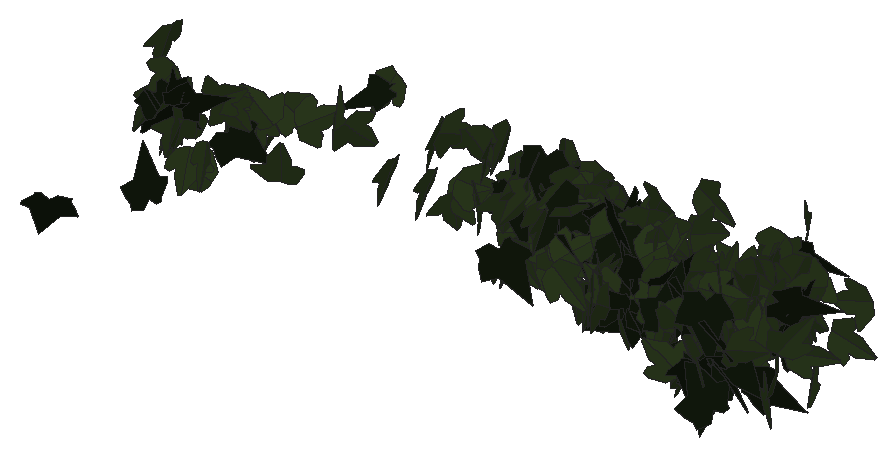
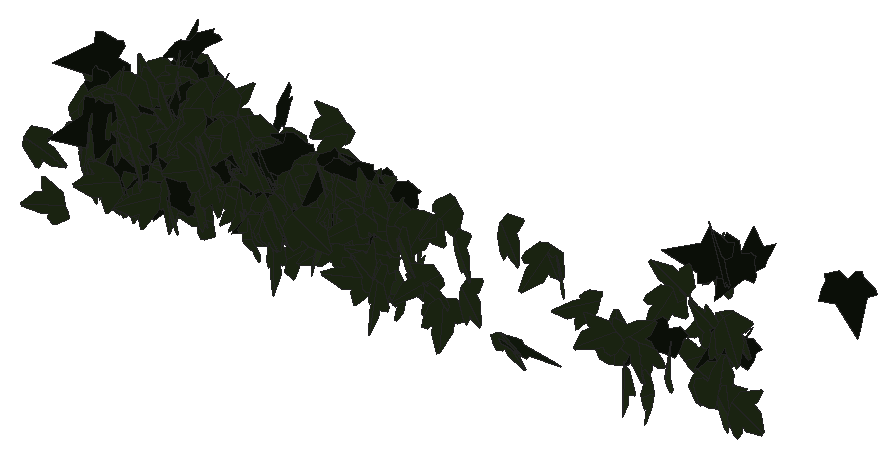
# SketchUp Ruby script. Lengths in inches.
U = 1.inch
M = Sketchup.active_model
def pt(a) = Geom::Point3d.new(a.map { |v| v * U })
def face(e, loops, mat)
  f = e.add_face(loops[0].map { |a| pt(a) })
  loops[1..].each { |l| e.add_face(l.map { |a| pt(a) }).erase! }
  f.material = f.back_material = mat if mat
  f
end
# faces: each face lists its corners as indices into pts; further lists are holes
def faces(e, pts, list, mat = nil) = list.each { |f| face(e, (f[0].is_a?(Array) ? f : [f]).map { |l| l.map { |i| pts[i] } }, mat) }
# xy, xz, yz: faces in a plane at the given z, y or x. An outline is a flat list of corners, or four numbers for a rectangle; further outlines are holes
def ring(l) = l.size == 4 ? [[l[0], l[1]], [l[2], l[1]], [l[2], l[3]], [l[0], l[3]]] : l.each_slice(2).to_a
def flat(e, list, mat, &to3) = list.each { |f| face(e, (f[0].is_a?(Array) ? f : [f]).map { |l| ring(l).map { |u, v| to3.(u, v) } }, mat) }
def xy(e, z, list, mat = nil) = flat(e, list, mat) { |x, y| [x, y, z] }
def xz(e, y, list, mat = nil) = flat(e, list, mat) { |x, z| [x, y, z] }
def yz(e, x, list, mat = nil) = flat(e, list, mat) { |y, z| [x, y, z] }
def lines(e, pts, list) = list.each { |a, b| e.add_line(pt(pts[a]), pt(pts[b])) }
# prism: a flat outline (further loops are holes) pulled along v
def prism(e, loops, v, mat = nil)
  f = face(e, loops, mat); d = Geom::Vector3d.new(v.map { |x| x * U })
  f.pushpull(f.normal.samedirection?(d) ? d.length : -d.length)
end
def box(e, o, s, mat = nil) = prism(e, [[o, [o[0] + s[0], o[1], o[2]], [o[0] + s[0], o[1] + s[1], o[2]], [o[0], o[1] + s[1], o[2]]]], [0, 0, s[2]], mat)
def at(x, y, z, deg = 0) = Geom::Transformation.translation(pt([x, y, z])) * Geom::Transformation.rotation(ORIGIN, Z_AXIS, deg.degrees)
def axes(o, x, y, z) = Geom::Transformation.new([*x, 0, *y, 0, *z, 0, *pt(o).to_a, 1])
def part(name) = M.definitions.add(name)
# library, detail: a bought-in or finely detailed component or shape, given as its bounding box
def library(name, o, s) = part(name).tap { |d| box(d.entities, o, s) }
def detail(e, o, s) = box(e.add_group.entities, o, s)
def put(e, d, t, mat = nil) = e.add_instance(d, t).tap { |i| i.material = mat if mat }
def group(e, t, mat = nil) = e.add_group.tap { |g| g.transformation = t; g.material = mat if mat }.entities
root = M.entities
M.materials.add("efeu1").color = [18, 25, 13]
M.materials.add("efeu2").color = [43, 57, 29]
c1 = part("ivyleaf_10")
p = [[0,0.5,-0.03],[-0.0625,2.02,-0.43],[-0.19,2.01,-0.46],[-0.54,1.05,-0.29],[-0.52,0.625,-0.18],[-0.83,0.76,-0.28],
  [-1.16,0.64,-0.33],[-1.15,0.33,-0.24],[-0.77,-0.39,0.02],[-0.3,-0.51,0.16],[0.04,-0.48,0.23],[-0.02,2.01,-0.4375],
  [-0.06,2.01,-0.43],[0.04,-0.49,0.23],[0.67,-0.49,0.14],[1.38,0.36,-0.2],[1.375,0.51,-0.24],[0.81,0.65,-0.19],
  [0.62,0.59,-0.15],[0.6,1.09,-0.28],[0.5,1.23,-0.31]]
faces(c1.entities,p,[[0,1,2,3,4,5,6,7,8,9,10],[11,12,0,13,14,15,16,17,18,19,20]],"efeu2")
c2 = part("ivyleaf_9")
p = [[1.54,2.16,1.25],[1.36,2.04,1.19],[-0.21,0.99,0.68],[-0.71,1.11,0.82],[-0.85,0.86,0.67],[-0.8,0.17,0.21],
  [-0.9,-0.01,0.1],[-0.67,-0.16,-0.02],[-0.08,-0.08,-0.05],[-0.03,-0.6,-0.4],[0.65,-0.88,-0.66],[0.83,-0.6,-0.49],
  [1.29,-0.42,-0.43],[1.8125,-0.07,-0.26],[1.21,0.44,0.15]]
faces(c2.entities,p,[[0,1,2,3,4,5,6,7,8,9,10,11,12,13,14]],"efeu1")
put(root,c1,axes([5.51,225.25,196.43],[-0.00871,-0.39501,0.30641],[-0.00096,-0.30645,-0.39508],[0.49992,-0.00747,0.00458]))
put(root,c1,axes([6.01,225.07,198.33],[-0.03947,-0.49188,0.0806],[-0.00697,-0.0803,-0.49346],[0.49839,-0.04008,-0.00052]))
put(root,c1,axes([6.17,225.02,196.24],[0.21308,-0.40089,0.20948],[0.09298,-0.18779,-0.45397],[0.44266,0.23242,-0.00548]))
put(root,c1,axes([6.45,224.92,196.28],[-0.3034,-0.37495,-0.13174],[-0.08173,-0.10333,0.48233],[-0.38893,0.31422,0.00141]))
put(root,c1,axes([6.75,224.14,197.875],[0.40554,-0.13098,-0.2615],[-0.24899,0.07991,-0.42617],[0.15343,0.47588,-0.00041]))
put(root,c2,axes([6.83,224.3125,196.54],[0.08787,-0.42556,0.04033],[0.00079,0.03961,0.45052],[-0.46151,-0.08096,0.00845]))
put(root,c1,axes([6.97,224.68,196.51],[-0.19663,-0.29472,0.35281],[-0.15437,-0.31912,-0.35261],[0.43302,-0.24759,0.03451]))
put(root,c2,axes([6.57,223.96,197.34],[-0.0252,-0.08588,-0.44283],[0.17951,0.3922,-0.09173],[0.43342,-0.16743,0.01225]))
put(root,c2,axes([7.02,219.33,196.69],[0.20864,0.29118,-0.26944],[-0.16333,-0.2105,-0.36332],[-0.38795,0.24522,0.00806]))
put(root,c1,axes([6.97,224.1,197.32],[-0.0102,-0.49375,-0.07812],[0.00657,0.078,-0.49384],[0.49985,-0.0111,0.00489]))
put(root,c1,axes([7.25,224.01,197.37],[0.12864,-0.06027,-0.4794],[0.42719,-0.21759,0.14198],[-0.22574,-0.44612,-0.00448]))
put(root,c1,axes([7.5625,225.34,196.7],[0.02039,-0.02319,0.49905],[0.37881,-0.32491,-0.03058],[0.32571,0.37933,0.00431]))
put(root,c1,axes([7.71,225.85,196.34],[-0.18336,0.23066,-0.40395],[0.2374,-0.32699,-0.29448],[-0.40002,-0.29979,0.0104]))
put(root,c1,axes([8.3125,223.46,195.99],[0.1796,0.16788,0.37983],[-0.33328,-0.19995,0.24171],[0.27818,-0.34794,0.04436]))
put(root,c2,axes([7.89,222.85,198.08],[-0.06625,0.19041,0.40172],[0.12801,-0.36764,0.20805],[0.44714,0.13346,-0.00004]))
put(root,c2,axes([8.16,221.94,198.16],[0.19304,0.37452,0.13565],[0.04989,0.12244,-0.43144],[-0.42539,0.18431,0.01096]))
put(root,c1,axes([8.27,222.95,196.7],[0.31926,0.30758,-0.08848],[-0.06341,-0.06158,-0.44366],[-0.33877,0.30138,-0.00035]))
put(root,c1,axes([8.58,222.26,197.95],[-0.24716,-0.34065,0.15004],[-0.07763,-0.12546,-0.42668],[0.39192,-0.23968,0.01011]))
put(root,c1,axes([8.59,225.64,196.43],[0.10853,-0.33026,-0.35937],[-0.10802,0.34277,-0.34762],[0.47598,0.15309,0.00306]))
put(root,c2,axes([8.28,222.58,198.23],[0.17719,0.03522,0.41738],[0.42368,0.08467,-0.17452],[-0.09903,0.42523,0.00018]))
put(root,c1,axes([8.55,225.1,196.875],[0.49276,0.05511,0.0644],[0.06364,0.01033,-0.49583],[-0.05598,0.49685,0.00317]))
put(root,c1,axes([8.91,225.1,197.08],[0.29884,0.17796,0.29598],[-0.27991,-0.1211,0.34081],[0.23035,-0.37801,0.03016]))
put(root,c1,axes([8.47,223.77,197.96],[-0.26011,-0.09677,0.36304],[0.34862,0.13289,0.26993],[-0.17754,0.40274,-0.00184]))
put(root,c1,axes([8.57,222.22,197.98],[0.01233,-0.02923,0.45122],[0.28144,-0.34699,-0.03144],[0.37597,0.26071,0.00874]))
put(root,c1,axes([8.66,223.95,197.74],[-0.27461,-0.26042,-0.24775],[0.20071,0.15082,-0.37776],[0.32406,-0.3141,0.02403]))
put(root,c2,axes([8.625,224.09,196.93],[0.02084,-0.10814,-0.43774],[0.03487,0.42051,-0.11083],[0.46804,-0.02651,0.02775]))
put(root,c1,axes([8.79,222.86,197.07],[0.37105,-0.21446,0.16508],[0.14114,-0.09036,-0.42114],[0.25123,0.36751,-0.00721]))
put(root,c2,axes([8.99,220.5625,196.96],[-0.2093,-0.30201,0.25572],[0.2096,0.16322,0.36758],[-0.36465,0.26716,0.06451]))
put(root,c1,axes([9.24,225.47,197.22],[0.22256,0.14028,0.42519],[0.36667,0.21538,-0.26299],[-0.25694,0.42888,-0.007]))
put(root,c1,axes([9.8125,224.48,196.09],[-0.45329,-0.211,0.00226],[0.01078,-0.01782,0.49957],[-0.21074,0.45295,0.02071]))
put(root,c2,axes([10.63,227.4,197.375],[-0.44825,0.13023,-0.00172],[-0.06384,-0.19329,-0.4006],[-0.12534,-0.36729,0.2102]))
put(root,c1,axes([10.21,224.91,197.43],[0.14469,-0.02283,-0.47806],[0.27982,0.40922,0.06514],[0.38829,-0.28639,0.13119]))
put(root,c1,axes([10.63,227.63,197.48],[-0.42018,0.16021,0.11484],[-0.20266,-0.24368,-0.31993],[-0.05556,-0.32277,0.29854]))
put(root,c1,axes([11.23,224.79,197.64],[0.38899,-0.24839,0.19233],[-0.16135,0.10468,0.46153],[-0.26954,-0.42112,0.00129]))
put(root,c1,axes([11.79,224.59,198.03],[-0.21625,-0.30705,-0.33009],[0.17888,0.2776,-0.37542],[0.41381,-0.28046,-0.01021]))
put(root,c1,axes([13.4,225.53,196.8],[0.1326,-0.4402,0.19658],[0.06565,-0.18549,-0.45966],[0.47761,0.14771,0.0086]))
put(root,c1,axes([13.47,224,197.82],[0.11382,-0.46952,0.12885],[0.02854,-0.12566,-0.48311],[0.48604,0.11733,-0.0018]))
put(root,c1,axes([13.5625,225.61,198.11],[0.22346,-0.43884,0.08652],[0.03641,-0.07854,-0.49245],[0.4458,0.22639,-0.00314]))
put(root,c1,axes([13.92,225.77,196.35],[-0.20323,-0.44838,-0.08746],[0.03872,0.07847,-0.49228],[0.45519,-0.20687,0.00282]))
put(root,c1,axes([14.27,225.05,198.57],[-0.09208,-0.20669,-0.44587],[0.18007,0.40789,-0.22627],[0.45727,-0.20224,-0.00068]))
put(root,c1,axes([14.08,225.74,196.45],[0.22099,-0.10158,-0.43686],[0.433,-0.07865,0.23733],[-0.11693,-0.48321,0.05321]))
put(root,c1,axes([14.4,225.67,196.95],[0.10242,0.22337,0.43545],[0.18932,0.39216,-0.24569],[-0.4513,0.21521,-0.00425]))
put(root,c1,axes([14.61,225.6,198.35],[-0.43512,-0.15244,-0.19348],[0.18193,0.06589,-0.46104],[0.16605,-0.47162,-0.00187]))
put(root,c1,axes([14.76,226.16,197.97],[0.23406,-0.41999,0.13722],[0.0573,-0.12512,-0.48069],[0.4381,0.24074,-0.01044]))
put(root,c1,axes([15.01,225.34,196.59],[-0.21854,0.17717,0.41334],[0.32182,-0.25939,0.28133],[0.31412,0.38901,-0.00067]))
put(root,c1,axes([15.15,226.1,198.29],[0.06769,-0.21967,0.44403],[0.24565,-0.37429,-0.22262],[0.4302,0.24829,0.05726]))
put(root,c1,axes([15.74,225.95,196.27],[0.06599,-0.36692,-0.33319],[-0.03691,0.33155,-0.37244],[0.49425,0.07375,0.01667]))
put(root,c1,axes([15.92,224.82,195.6],[0.19313,-0.20897,0.41113],[-0.24556,0.33069,0.28344],[-0.39038,-0.3114,0.0251]))
put(root,c1,axes([16.13,225.12,196.15],[-0.00369,-0.34684,-0.36012],[0.00589,0.36008,-0.34685],[0.49995,-0.0068,0.00143]))
put(root,c1,axes([16.34,225.35,197.76],[0.3431,0.096,-0.35081],[-0.33896,-0.09043,-0.35627],[-0.13185,0.48229,0.00303]))
put(root,c1,axes([15.875,226.04,196.77],[-0.04303,-0.08521,0.4908],[0.48162,-0.13294,0.01914],[0.12724,0.47441,0.09352]))
put(root,c1,axes([16.3,224.76,197.61],[-0.26457,-0.42416,0.00945],[-0.003,-0.00926,-0.49991],[0.42425,-0.26458,0.00235]))
put(root,c1,axes([16.26,225.11,196.18],[0.14622,-0.43523,0.19798],[0.06137,-0.18823,-0.45913],[0.47419,0.15856,-0.00163]))
put(root,c2,axes([16.27,225.02,197.7],[-0.25706,-0.13592,-0.40675],[0.35385,0.20071,-0.2907],[0.2423,-0.43731,-0.007]))
put(root,c1,axes([16.11,225.37,197.96],[-0.01761,0.00755,0.49963],[0.49022,0.09712,0.01581],[-0.09681,0.49042,-0.01082]))
put(root,c1,axes([16.1875,224.98,196.63],[0.07241,-0.03655,-0.49338],[0.47782,0.13441,0.06017],[0.12823,-0.48021,0.0544]))
put(root,c1,axes([16.93,224.97,197.85],[-0.24297,-0.09258,0.42707],[-0.39508,-0.16228,-0.25995],[0.18674,-0.46378,0.0057]))
put(root,c1,axes([16.59,225.03,198.07],[-0.01284,0.0372,0.49845],[0.16633,-0.46988,0.03936],[0.47135,0.16683,-0.00031]))
put(root,c1,axes([16.87,224.9375,197.89],[-0.05664,-0.23747,0.43635],[-0.00745,-0.43872,-0.23972],[0.49673,-0.03366,0.04616]))
put(root,c1,axes([16.68,225.29,198.24],[-0.03104,-0.08818,-0.49118],[0.1105,-0.48113,0.07939],[-0.48665,-0.10363,0.04936]))
put(root,c1,axes([16.48,224.71,196.22],[0.24281,0.00455,0.43706],[0.43119,0.07932,-0.24038],[-0.07153,0.49365,0.0346]))
put(root,c1,axes([16.98,226.12,198.55],[-0.0819,0.41566,-0.26555],[0.05152,-0.26051,-0.42365],[-0.49055,-0.09676,-0.00016]))
put(root,c1,axes([16.96,225.08,197.31],[-0.13015,-0.13295,-0.46409],[0.33411,0.32215,-0.18599],[0.34847,-0.35853,0.00498]))
put(root,c1,axes([16.8,225.2,195.93],[-0.06932,-0.03289,-0.49408],[0.49508,0.00481,-0.06979],[0.00934,-0.49889,0.0319]))
put(root,c1,axes([17.45,226.67,197.83],[-0.23217,-0.26893,0.35181],[-0.23339,-0.26328,-0.35527],[0.37634,-0.32918,-0.00328]))
put(root,c1,axes([16.97,224.92,197.82],[0.29802,0.18674,-0.35541],[0.30949,0.17508,0.35151],[0.25573,-0.42951,-0.01123]))
put(root,c2,axes([17.14,225.19,198.78],[-0.31106,-0.29201,-0.26071],[0.18792,0.18073,-0.42664],[0.3434,-0.36341,-0.00269]))
put(root,c1,axes([17.36,224.81,197.79],[-0.20524,-0.40096,-0.21704],[0.12179,0.18115,-0.44984],[0.43937,-0.23751,0.02331]))
put(root,c1,axes([17.6,224.5625,197.68],[0.15577,-0.46243,0.10907],[0.03184,-0.10436,-0.48795],[0.47405,0.15896,-0.00307]))
put(root,c1,axes([17.27,224.92,197.64],[-0.10569,0.00805,0.48864],[0.47912,-0.09681,0.10523],[0.0963,0.49047,0.01274]))
put(root,c1,axes([17.6,225.82,197.86],[0.04412,0.44839,-0.2168],[-0.04427,-0.21326,-0.45007],[-0.49608,0.05891,0.02089]))
put(root,c2,axes([17.45,223.12,197.33],[-0.13327,-0.18236,-0.44608],[0.28742,0.34142,-0.22544],[0.38682,-0.31651,0.01383]))
put(root,c1,axes([17.55,225.25,196.63],[-0.2795,-0.11951,-0.39699],[0.37384,0.13434,-0.30364],[0.17924,-0.46655,0.01426]))
put(root,c1,axes([17.65,225.83,196.4],[-0.25272,0.10479,0.41851],[0.2943,-0.31279,0.25603],[0.31547,0.37574,0.09642]))
put(root,c1,axes([17.85,225.38,198.5],[0.26738,-0.4213,-0.03191],[-0.01707,0.02696,-0.49898],[0.42216,0.26792,0.00003]))
put(root,c1,axes([17.46,224.76,196.08],[0.01337,0.02183,0.49934],[0.44926,0.2184,-0.02157],[-0.21905,0.44925,-0.01377]))
put(root,c2,axes([17.93,224.77,198.33],[0.0026,0.08912,-0.49199],[-0.26958,0.4146,0.07368],[0.42109,0.26488,0.05021]))
put(root,c1,axes([18.14,224.9,198.66],[0.15487,0.2117,-0.42568],[-0.26969,-0.32956,-0.26202],[-0.39151,0.31076,0.01211]))
put(root,c1,axes([17.83,225.24,198.16],[-0.11392,-0.07441,-0.48113],[0.46672,0.12393,-0.12967],[0.13855,-0.47865,0.04122]))
put(root,c1,axes([18.33,225.14,198.35],[-0.3752,-0.32808,0.03987],[-0.02957,-0.02675,-0.49841],[0.32917,-0.37636,0.00067]))
put(root,c1,axes([18.45,226.23,197.6875],[0.28986,-0.20152,-0.35408],[-0.28812,0.20583,-0.35301],[0.28804,0.40869,0.00321]))
put(root,c2,axes([18.01,224.67,197.52],[-0.01801,-0.00105,-0.49967],[0.46053,-0.19403,-0.01619],[-0.19387,-0.46082,0.00795]))
put(root,c1,axes([18.05,224.84,197.125],[0.41863,0.16787,0.2158],[0.2023,0.07527,-0.45101],[-0.18391,0.46492,-0.00491]))
put(root,c1,axes([18.55,226.25,197.65],[0.23083,-0.17369,-0.40811],[-0.31587,0.2586,-0.28872],[0.31136,0.3911,0.00966]))
put(root,c2,axes([18.47,224.62,198.31],[-0.43603,-0.24087,0.0431],[-0.03375,-0.02802,-0.49807],[0.24236,-0.43726,0.00817]))
put(root,c1,axes([18.41,225.6875,198.15],[0.05481,-0.46679,0.17059],[0.03951,-0.16699,-0.46963],[0.49541,0.06496,0.01858]))
put(root,c1,axes([18.15,224.49,197.8],[0.28101,0.0175,-0.41319],[0.37212,0.20728,0.26185],[0.18046,-0.45468,0.10347]))
put(root,c1,axes([18.46,224.49,198.11],[-0.39117,-0.29295,-0.10564],[0.08619,0.06114,-0.48871],[0.29925,-0.40055,0.00267]))
put(root,c1,axes([18.6,225.54,196.07],[-0.01903,0.06901,-0.49485],[-0.10857,-0.48395,-0.06331],[-0.4877,0.10504,0.0334]))
put(root,c1,axes([18.55,225.39,197.9],[-0.12656,-0.18207,-0.44814],[0.22901,0.38547,-0.22128],[0.42607,-0.26127,-0.01418]))
put(root,c1,axes([18.8,225.94,196.29],[0.08414,-0.43954,-0.22299],[-0.05202,0.21703,-0.44743],[0.49012,0.0985,-0.00921]))
put(root,c1,axes([18.91,224.19,196.25],[-0.45854,0.11048,0.16595],[-0.16491,0.02367,-0.47143],[-0.11202,-0.48707,0.01473]))
put(root,c1,axes([18.54,224.91,196.75],[0.43391,0.05844,-0.24147],[0.23435,0.06502,0.43687],[0.08246,-0.4923,0.02904]))
put(root,c1,axes([18.79,226.32,197.29],[0.40046,0.26953,-0.13034],[-0.10799,-0.07298,-0.48271],[-0.27923,0.41476,-0.00023]))
put(root,c2,axes([18.83,224.5,197.1],[0.2713,-0.41862,-0.03393],[0.0203,-0.02727,0.49884],[-0.4195,-0.27205,0.0022]))
put(root,c1,axes([18.83,224.92,196.99],[-0.07592,0.07261,0.48884],[0.16361,-0.46299,0.09418],[0.46634,0.17425,0.04654]))
put(root,c1,axes([18.88,225.68,197.43],[-0.34667,-0.29834,-0.20202],[0.15177,0.13334,-0.45737],[0.32678,-0.37843,-0.0019]))
put(root,c1,axes([18.91,226.21,196.9375],[-0.08821,0.25269,0.42234],[0.10664,-0.40906,0.26702],[0.48047,0.13718,0.01827]))
put(root,c2,axes([18.73,225.67,197.31],[0.03102,-0.06419,-0.49489],[0.23073,0.44151,-0.04281],[0.4425,-0.22571,0.05701]))
put(root,c2,axes([19.17,225.61,196.55],[0.15922,-0.35697,0.3118],[-0.10369,0.29472,0.39037],[-0.46249,-0.18898,0.01982]))
put(root,c1,axes([18.75,223.81,197.36],[0.29044,0.01371,-0.40676],[0.38311,0.15946,0.27893],[0.13737,-0.47369,0.08212]))
put(root,c1,axes([19.35,225.9,196.59],[0.10372,0.22432,0.43465],[-0.20542,-0.38325,0.24682],[0.4439,-0.22978,0.01265]))
put(root,c1,axes([18.85,226.7,196.91],[0.22689,-0.07898,0.4385],[0.40354,-0.17219,-0.23981],[0.18889,0.46272,-0.0144]))
put(root,c1,axes([18.98,225.71,196.58],[-0.00841,-0.09255,0.49129],[0.40869,-0.28426,-0.04655],[0.28792,0.40079,0.08043]))
put(root,c2,axes([18.99,224.65,198.04],[0.15749,0.26413,-0.39425],[0.16626,0.35835,0.30649],[0.44447,-0.22764,0.02504]))
put(root,c1,axes([19.36,224.66,196.29],[0.01902,-0.09521,-0.49048],[0.01257,0.49077,-0.09478],[0.49948,-0.00872,0.02106]))
put(root,c1,axes([19.18,224.23,196.19],[0.00344,-0.13409,0.48167],[0.32919,-0.36194,-0.10312],[0.37633,0.31783,0.08579]))
put(root,c1,axes([19.08,224.7,196.78],[-0.18379,-0.05931,-0.4612],[0.45386,0.08501,-0.19179],[0.10117,-0.48914,0.02259]))
put(root,c2,axes([19.51,225.51,198.22],[-0.37467,0.13579,-0.30197],[0.2846,-0.10094,-0.39851],[-0.16919,-0.4705,-0.00165]))
put(root,c1,axes([19.5,224.66,196.29],[0.49764,0.03516,-0.03348],[-0.03375,0.00275,-0.49885],[-0.0349,0.49875,0.00511]))
put(root,c1,axes([19.58,225.48,197.53],[0.47741,-0.06102,-0.13548],[0.13503,-0.01214,0.48127],[-0.06202,-0.49611,0.00489]))
put(root,c1,axes([19.9,224.59,196.42],[0.44856,-0.01743,-0.22021],[-0.22008,0.00756,-0.4489],[0.01898,0.49964,-0.00089]))
put(root,c1,axes([19.52,225.03,197.02],[0.36785,-0.11044,-0.32014],[0.32173,-0.03357,0.38126],[-0.10571,-0.48649,0.04637]))
put(root,c1,axes([19.53,224.27,198.05],[0.09741,0.0382,-0.48893],[0.41758,0.25493,0.10312],[0.25717,-0.42843,0.01776]))
put(root,c2,axes([19.94,224.57,198.22],[-0.42989,-0.25532,-0.00099],[0.00369,-0.00426,-0.49997],[0.2553,-0.42987,0.00555]))
put(root,c1,axes([19.89,225.67,196.82],[0.01362,0.42957,-0.25551],[-0.00676,0.25574,0.4296],[0.49977,-0.00825,0.01277]))
put(root,c1,axes([20.04,224.97,196.54],[0.30968,-0.22458,-0.32197],[-0.25933,0.19083,-0.38254],[0.2947,0.40392,0.00171]))
put(root,c1,axes([19.875,224.26,197.31],[0.0826,-0.39128,0.30013],[0.05644,-0.29481,-0.39988],[0.48989,0.09994,-0.00454]))
put(root,c1,axes([20.1875,224.74,196.29],[0.26039,-0.02006,-0.42638],[-0.42334,0.05177,-0.26097],[0.05462,0.49691,0.00997]))
put(root,c1,axes([19.75,224,197.02],[-0.23635,0.21768,0.38309],[0.28258,-0.25866,0.32131],[0.33807,0.36839,-0.00075]))
put(root,c2,axes([20.32,223.89,196.69],[-0.3101,0.16121,0.35756],[-0.3173,0.16483,-0.3495],[-0.23056,-0.44367,0.00008]))
put(root,c1,axes([19.7,223.66,196.96],[0.20765,-0.18455,0.41572],[0.3186,-0.26714,-0.27773],[0.32462,0.38024,0.00666]))
put(root,c1,axes([19.74,225.03,196.73],[-0.3619,-0.03888,0.3428],[0.34309,0.01168,0.36353],[-0.03627,0.49835,0.01823]))
put(root,c1,axes([20.14,223.92,196.86],[0.19195,0.35365,0.2968],[-0.14038,-0.2615,0.40238],[0.43983,-0.2378,-0.0011]))
put(root,c1,axes([19.72,222.39,197.8125],[0.29168,0.10157,0.3932],[0.37297,0.12455,-0.30884],[-0.16068,0.47347,-0.00311]))
put(root,c1,axes([19.83,225.76,196.46],[0.06403,-0.13925,-0.47593],[0.24514,-0.40825,0.15243],[-0.43105,-0.25286,0.01599]))
put(root,c2,axes([20.04,223.92,198.93],[0.37048,-0.16522,-0.2923],[-0.26769,0.11742,-0.40565],[0.20269,0.45707,-0.00145]))
put(root,c1,axes([20.39,225.39,198.65],[-0.39591,0.05316,0.30072],[-0.29856,0.03611,-0.39945],[-0.06418,-0.49585,0.00315]))
put(root,c1,axes([20.15,223.41,196.75],[0.00813,-0.29174,-0.40598],[0.05678,0.40395,-0.28914],[0.4967,-0.0414,0.03969]))
put(root,c2,axes([20.17,224.63,197.79],[0.39703,0.27857,-0.12152],[-0.09819,-0.07164,-0.485],[-0.28763,0.40898,-0.00218]))
put(root,c2,axes([20.35,224.55,197.1],[-0.02104,-0.43283,0.24943],[0.03592,0.24769,0.43285],[-0.49826,0.03613,0.02067]))
put(root,c1,axes([20.43,224.89,198.55],[-0.40873,-0.2678,0.10595],[-0.08704,-0.06048,-0.48864],[0.27453,-0.41788,0.00283]))
put(root,c2,axes([20.64,223.83,196.54],[0.02799,0.03717,-0.49783],[-0.39461,-0.30376,-0.04487],[-0.30578,0.39541,0.01233]))
put(root,c1,axes([20.5,223.84,196.23],[-0.22796,0.34487,0.28126],[-0.1548,0.23482,-0.4134],[-0.41722,-0.27555,-0.00029]))
put(root,c1,axes([20.5,225.04,196.58],[0.12603,0.30297,-0.37727],[0.15302,0.34489,0.32808],[0.45902,-0.19815,-0.00579]))
put(root,c1,axes([20.48,224.6875,196.53],[0.33998,0.35708,0.08312],[0.05737,0.06014,-0.49304],[-0.36211,0.34479,-0.00008]))
put(root,c1,axes([20.93,224.93,198],[0.20864,0.07608,0.44797],[-0.44207,-0.08003,0.21948],[0.1051,-0.48765,0.03387]))
put(root,c1,axes([20.45,224.87,197.78],[0.25646,-0.2875,-0.31871],[0.20341,-0.24552,0.38516],[-0.37796,-0.32721,-0.00897]))
put(root,c1,axes([20.49,226.87,198.25],[0.1951,-0.00281,0.46036],[0.45384,0.08507,-0.19182],[-0.07725,0.4927,0.03575]))
put(root,c1,axes([20.58,224.59,196.5625],[0.01097,-0.11273,-0.487],[0.42374,0.26052,-0.05076],[0.26519,-0.41161,0.10125]))
put(root,c2,axes([20.69,224.3125,196.32],[0.1985,-0.45711,0.04064],[0.02304,-0.0343,-0.49829],[0.45833,0.19969,0.00745]))
put(root,c1,axes([20.71,224.53,197.82],[0.23448,0.04645,-0.43916],[0.32187,0.32246,0.20596],[0.30235,-0.3793,0.12131]))
put(root,c1,axes([21.04,224.36,196.7],[-0.38004,0.31315,0.08663],[-0.07013,0.05111,-0.49241],[-0.31725,-0.38643,0.00508]))
put(root,c1,axes([20.92,224.86,198.32],[-0.28815,-0.31191,-0.26397],[0.19114,0.1826,-0.42441],[0.36116,-0.3455,0.014]))
put(root,c2,axes([20.93,224.3125,196.29],[-0.26406,0.36978,0.20865],[0.11859,-0.1717,0.45438],[0.40769,0.28945,0.00297]))
put(root,c1,axes([20.85,225.61,197.14],[-0.35006,0.11952,-0.33641],[0.3154,-0.11724,-0.36984],[-0.16729,-0.47114,0.00669]))
put(root,c1,axes([21.07,225.8,198.04],[0.38673,-0.31059,0.06302],[0.05222,-0.03562,-0.49599],[0.31259,0.39021,0.00489]))
put(root,c1,axes([21.3,224.47,197.59],[0.29868,0.35265,-0.19086],[-0.13122,-0.13892,-0.46204],[-0.37891,0.32609,0.00957]))
put(root,c1,axes([21.25,225.61,196.57],[0.17116,-0.41068,0.22814],[0.11163,-0.20031,-0.44432],[0.45634,0.20303,0.02312]))
put(root,c2,axes([21.23,224.54,197.08],[0.3317,0.36516,0.08146],[-0.06238,-0.05336,0.49322],[0.36889,-0.33736,0.01016]))
put(root,c1,axes([21.51,225.33,196.68],[0.2867,-0.40509,-0.06087],[-0.03538,0.04953,-0.49628],[0.40811,0.28888,-0.00026]))
put(root,c1,axes([21.29,225.26,197.19],[0.1356,-0.14539,-0.45877],[0.28298,-0.36145,0.19819],[-0.38928,-0.31339,-0.01573]))
put(root,c1,axes([21.22,225.44,196.05],[0.08094,-0.03366,0.49226],[0.4909,0.05567,-0.07691],[-0.04963,0.49575,0.04205]))
put(root,c1,axes([21.66,225.24,198.32],[-0.02404,0.15402,0.47508],[-0.0615,0.47109,-0.15585],[-0.49562,-0.06593,-0.00371]))
put(root,c1,axes([21.33,224.53,196.93],[0.17086,-0.02668,0.46914],[0.46505,-0.06192,-0.1729],[0.06733,0.49543,0.00366]))
put(root,c1,axes([21.85,223.97,196.46],[0.18844,-0.37251,-0.27518],[-0.12101,0.24716,-0.41745],[0.44704,0.22393,0.00299]))
put(root,c2,axes([21.53,225.51,196.39],[-0.21171,0.07187,0.44723],[0.42303,-0.14512,0.22358],[0.16194,0.47305,0.00064]))
put(root,c1,axes([21.75,223.55,197.03],[0.48904,-0.09939,0.03105],[0.03088,-0.00392,-0.49903],[0.09944,0.49001,0.00231]))
put(root,c1,axes([21.5,225.52,197.3],[0.00085,-0.01393,0.49981],[0.41973,0.27163,0.00686],[-0.27172,0.41955,0.01215]))
put(root,c1,axes([21.75,224.09,196.12],[-0.03536,0.04315,0.49688],[0.25363,-0.42735,0.05516],[0.42944,0.25595,0.00833]))
put(root,c2,axes([21.95,223.73,196.79],[-0.33175,-0.15841,0.33889],[0.30666,0.14426,0.36763],[-0.21425,0.45177,0.00144]))
put(root,c1,axes([21.84,224.99,197.78],[-0.38267,-0.19011,-0.25966],[0.22683,0.12685,-0.42715],[0.22829,-0.44471,-0.01084]))
put(root,c1,axes([22.04,224.12,197.25],[0.259,-0.40364,0.14139],[0.07351,-0.12083,-0.47958],[0.42132,0.26921,-0.00324]))
put(root,c1,axes([21.96,226.56,196.82],[0.02444,0.02413,-0.49882],[0.25292,0.43004,0.03319],[0.43062,-0.25394,0.00882]))
put(root,c2,axes([22.05,224.39,197.22],[0.00205,-0.38764,0.3158],[-0.00569,-0.3158,-0.38761],[0.49996,-0.00201,-0.00571]))
put(root,c1,axes([22.26,225.53,196.52],[0.0366,-0.4825,-0.12592],[-0.00708,0.12574,-0.48388],[0.49861,0.03721,0.00237]))
put(root,c1,axes([22.13,225.58,196.1],[0.18832,-0.22431,0.40524],[0.28453,-0.28917,-0.29228],[0.36549,0.34069,0.01873]))
put(root,c2,axes([22.46,225.36,196.53],[-0.05291,0.21696,-0.44736],[0.097,-0.43674,-0.22328],[-0.48764,-0.11041,0.00413]))
put(root,c1,axes([22.41,225.43,197.65],[-0.09836,0.0311,0.48924],[0.08605,-0.49015,0.04846],[0.48262,0.09373,0.09107]))
put(root,c1,axes([22.57,225.28,196.9],[-0.17007,-0.46505,0.06928],[-0.02473,-0.06472,-0.49518],[0.46954,-0.17186,-0.00099]))
put(root,c1,axes([22.54,223.96,198.25],[-0.04789,-0.23351,-0.43952],[0.12892,0.42066,-0.23753],[0.48072,-0.13607,0.01992]))
put(root,c1,axes([22.63,226.4,197.77],[0.28275,-0.41086,0.03535],[0.02294,-0.02712,-0.49874],[0.41174,0.28366,0.00351]))
put(root,c1,axes([22.52,224.46,195.97],[0.00762,-0.00766,0.49988],[0.31343,0.38957,0.00119],[-0.38949,0.31333,0.01074]))
put(root,c1,axes([22.65,223.39,195.91],[-0.04484,0.06723,0.49343],[0.28323,-0.40405,0.08079],[0.4096,0.28675,-0.00185]))
put(root,c2,axes([23.15,225.23,196.875],[-0.17697,-0.23404,-0.40485],[-0.21448,-0.34404,0.29264],[-0.41555,0.27724,0.02137]))
put(root,c1,axes([22.71,223.63,196.94],[-0.35863,0.02568,0.34745],[0.33389,-0.11707,0.35328],[0.0995,0.48542,0.06683]))
put(root,c2,axes([22.74,223.54,196.32],[-0.22668,-0.24241,-0.37397],[0.27764,0.25138,-0.33124],[0.34861,-0.35783,0.02064]))
put(root,c1,axes([22.78,224.78,197.74],[0.44217,-0.20739,-0.10714],[0.0977,-0.04401,0.48838],[-0.212,-0.45283,0.00161]))
put(root,c2,axes([22.625,224.97,197.02],[0.01803,0.00389,-0.49966],[0.49791,-0.0421,0.01763],[-0.04194,-0.49821,-0.00539]))
put(root,c2,axes([23.05,223.36,197.08],[0.07085,-0.46171,0.17835],[-0.00129,0.17999,0.46648],[-0.49495,-0.06656,0.02431]))
put(root,c1,axes([22.79,222.84,197.76],[-0.35297,-0.07123,-0.3469],[0.33959,0.07082,-0.36008],[0.10043,-0.48981,-0.00161]))
put(root,c1,axes([23.18,225.21,197.12],[0.13253,0.18929,-0.4434],[-0.2508,-0.36566,-0.23107],[-0.41175,0.28365,-0.00198]))
put(root,c2,axes([23.2,223.84,197.36],[0.19715,-0.09395,-0.44978],[-0.41352,0.17711,-0.21825],[0.20033,0.45805,-0.00786]))
put(root,c1,axes([22.91,225.94,195.93],[-0.32071,0.14608,0.35469],[0.3283,-0.13461,0.35228],[0.19841,0.45885,-0.00957]))
put(root,c2,axes([22.97,225.43,196.66],[-0.02204,-0.49906,0.02124],[0.00076,-0.02129,-0.49955],[0.49951,-0.02198,0.00169]))
put(root,c1,axes([22.95,224.75,196.14],[-0.13714,0.26793,-0.39926],[0.17192,-0.36041,-0.30091],[-0.44904,-0.21981,0.00673]))
put(root,c1,axes([23.03,224.24,196.68],[-0.30266,-0.35811,0.17366],[0.11232,0.13245,0.46887],[-0.38181,0.32283,0.00028]))
put(root,c1,axes([23.25,225.51,196.69],[-0.07864,-0.37796,0.31775],[-0.08551,-0.30647,-0.3857],[0.48632,-0.115,-0.01644]))
put(root,c1,axes([23.22,225.72,197.88],[-0.05397,-0.45561,0.19876],[-0.03555,-0.19588,-0.45866],[0.49581,-0.06364,-0.01125]))
put(root,c1,axes([22.84,223.7,197.95],[-0.2355,0.07996,-0.43376],[0.40426,-0.15752,-0.24852],[-0.17639,-0.46775,0.00954]))
put(root,c1,axes([23.32,222.17,196.74],[0.19952,0.33745,0.31035],[-0.15527,-0.26873,0.39201],[0.43137,-0.25281,-0.00244]))
put(root,c1,axes([23.41,227.01,198.31],[0.04238,-0.10149,-0.48775],[-0.16901,0.45756,-0.10989],[0.46866,0.17418,0.00447]))
put(root,c1,axes([23.44,225.95,198.125],[-0.00314,-0.47598,-0.15308],[-0.00099,0.15309,-0.47599],[0.49999,-0.00268,-0.00191]))
put(root,c1,axes([23.54,225.83,198.5],[0.45114,-0.09296,-0.19451],[-0.18768,0.05262,-0.46044],[0.10608,0.48846,0.01259]))
put(root,c2,axes([23.13,224.1,197.86],[0.24057,-0.35988,0.25023],[0.14604,-0.20333,-0.43282],[0.41328,0.28133,0.00728]))
put(root,c2,axes([23.51,224.53,197.71],[-0.39763,-0.23003,-0.19743],[0.16844,0.10307,-0.45935],[0.25203,-0.43181,-0.00448]))
put(root,c2,axes([23.56,225.74,196.3125],[-0.34729,-0.18112,0.31078],[0.27554,0.14374,0.39168],[-0.23123,0.44332,-0.00003]))
put(root,c1,axes([23.46,224.75,197.41],[-0.17811,-0.31075,-0.34887],[0.16537,0.30726,-0.35811],[0.43695,-0.24295,-0.00668]))
put(root,c1,axes([23.62,225.8,197.62],[-0.06312,-0.28439,0.40637],[-0.05832,-0.40256,-0.29077],[0.49256,-0.0841,0.01765]))
put(root,c1,axes([23.3,226,197.61],[0.26989,0.31133,0.28326],[0.18851,0.21145,-0.41201],[-0.37633,0.32918,-0.00324]))
put(root,c1,axes([23.65,225.73,196.47],[-0.20503,-0.44892,0.0802],[-0.03015,-0.07439,-0.49351],[0.45503,-0.20721,0.00343]))
put(root,c1,axes([23.53,225.41,195.77],[-0.04798,-0.48497,0.11182],[0.00942,0.11143,0.48733],[-0.4976,0.04887,-0.00156]))
put(root,c1,axes([23.32,223.86,198.26],[0.05491,-0.05847,0.49352],[0.40845,-0.27755,-0.07833],[0.28311,0.41176,0.01728]))
put(root,c1,axes([23.29,223.57,198.17],[-0.09203,-0.09542,-0.48211],[0.47065,0.12411,-0.1144],[0.1415,-0.47486,0.06697]))
put(root,c1,axes([23.73,222.85,197.57],[0.40236,-0.23251,-0.18452],[-0.15879,0.09401,-0.4647],[0.25079,0.43255,0.00181]))
put(root,c1,axes([23.31,226.43,196.74],[-0.19616,0.03584,-0.45852],[0.4574,-0.03687,-0.19856],[-0.04804,-0.49735,-0.01832]))
put(root,c1,axes([23.46,224.82,196],[-0.04386,-0.08115,0.49142],[0.24083,0.42836,0.09223],[-0.43598,0.24478,0.00151]))
put(root,c1,axes([23.76,224.25,196.78],[0.45014,-0.12231,0.18003],[-0.1747,0.04363,0.46645],[-0.12981,-0.48284,-0.00345]))
put(root,c1,axes([23.75,223.68,197.25],[-0.00287,0.07614,0.49416],[0.05961,-0.49059,0.07594],[0.49643,0.05935,-0.00626]))
put(root,c2,axes([23.68,223.55,196.07],[0.04711,0.15757,0.47218],[-0.13117,-0.4536,0.16446],[0.48018,-0.13936,-0.0014]))
put(root,c2,axes([23.47,222.86,197.67],[0.46804,-0.12955,0.11897],[0.11586,-0.02739,-0.48562],[0.13234,0.48215,0.00438]))
put(root,c1,axes([23.71,223.48,197.84],[-0.17867,0.41499,-0.21415],[0.08512,-0.19651,-0.45182],[-0.45917,-0.19791,-0.00043]))
put(root,c1,axes([23.55,225.92,198.07],[0.11647,0.07485,0.48045],[0.29104,0.38504,-0.13054],[-0.38953,0.31007,0.04612]))
put(root,c2,axes([23.5,226.35,198.08],[0.4166,-0.02202,0.27561],[0.27463,-0.02466,-0.4171],[0.03196,0.49891,-0.00846]))
put(root,c1,axes([23.52,224.54,198.11],[0.0254,0.00111,0.49935],[0.47734,0.14675,-0.02461],[-0.14662,0.47798,0.0064]))
put(root,c1,axes([23.92,224.84,198.42],[-0.49302,-0.02021,-0.08074],[0.08095,-0.00378,-0.49339],[0.01934,-0.49958,0.007]))
put(root,c1,axes([24,225.27,196.85],[0.02848,-0.49881,-0.01941],[0.00028,0.01946,-0.49962],[0.49919,0.02845,0.00139]))
put(root,c1,axes([24.04,224.07,197.8],[-0.17596,-0.46419,0.05972],[-0.01471,-0.05828,-0.49637],[0.46778,-0.17644,0.00685]))
put(root,c1,axes([24.32,224.18,196.86],[0.07123,0.00126,-0.4949],[-0.46012,0.1843,-0.06576],[0.18225,0.46479,0.02741]))
put(root,c1,axes([23.98,225.69,196.3],[-0.16327,-0.42478,-0.20714],[-0.06919,-0.19531,0.45505],[-0.4675,0.17726,0.00499]))
put(root,c2,axes([23.89,222.84,196.4],[-0.09496,-0.48973,0.0338],[-0.01015,-0.03246,-0.49884],[0.4908,-0.09543,-0.00377]))
put(root,c1,axes([23.875,224.33,197.875],[-0.42299,0.08786,0.25172],[0.24704,-0.04836,0.43201],[0.10026,0.48984,-0.0025]))
put(root,c1,axes([24.31,225.92,196.43],[-0.12026,0.12153,-0.46986],[-0.32395,0.34035,0.17094],[0.36138,0.34553,-0.00312]))
put(root,c1,axes([23.875,222.06,197.54],[-0.28993,0.25072,-0.32106],[0.23954,-0.21381,-0.38328],[-0.32948,-0.37607,0.00387]))
put(root,c2,axes([24.22,221.93,197.23],[0.15226,0.40488,-0.25077],[-0.0908,-0.23377,-0.43256],[-0.46752,0.17727,0.00234]))
put(root,c1,axes([24.25,225.76,198.23],[-0.21998,-0.40096,0.20208],[-0.09384,-0.17901,-0.45733],[0.4391,-0.23913,0.0035]))
put(root,c1,axes([23.93,225.38,196.82],[0.37607,-0.2742,-0.18272],[0.15981,-0.09068,0.46501],[-0.28815,-0.40815,0.01944]))
put(root,c2,axes([24.03,222.53,198.52],[-0.07462,-0.47381,-0.14121],[0.0161,0.1404,-0.47961],[0.49414,-0.07613,-0.0057]))
put(root,c1,axes([23.94,225.26,198.3],[0.15424,-0.21086,0.42632],[0.32644,-0.27901,-0.2561],[0.3459,0.35734,0.05159]))
put(root,c1,axes([23.9,225.06,197.59],[-0.18495,-0.01058,-0.46442],[0.46446,-0.01301,-0.18467],[-0.00817,-0.49972,0.01464]))
put(root,c2,axes([24.28,222.73,197.6],[0.35268,-0.34636,-0.07518],[0.05466,-0.05164,0.49431],[-0.35018,-0.35689,0.00144]))
put(root,c1,axes([24.42,225.99,197.6875],[0.3652,0.28824,-0.18316],[-0.14244,-0.11516,-0.46524],[-0.31039,0.39199,-0.002]))
put(root,c2,axes([24.22,225.06,196.14],[-0.22418,0.10139,0.43527],[0.26823,-0.35899,0.22176],[0.35749,0.33294,0.10657]))
put(root,c1,axes([24.48,224.43,197.8125],[-0.09093,0.28276,0.40221],[-0.15168,0.37295,-0.29648],[-0.46768,-0.17594,0.01795]))
put(root,c1,axes([24.4,223.82,197.11],[0.22318,0.38745,-0.22377],[0.0941,0.20382,0.44677],[0.43742,-0.24153,0.01806]))
put(root,c2,axes([24.78,221.76,196.34],[-0.29497,-0.38606,0.11813],[0.07389,0.09221,0.48584],[-0.39691,0.30407,0.00265]))
put(root,c2,axes([24.28,222.73,196.92],[0.28835,-0.35433,0.20324],[0.1318,-0.15477,-0.45681],[0.38663,0.31702,0.00415]))
put(root,c2,axes([24.58,222.6875,197.28],[0.10253,-0.29377,-0.39139],[-0.07841,0.38486,-0.30941],[0.48305,0.12482,0.03285]))
put(root,c1,axes([24.78,225.68,197.84],[-0.00917,0.18363,0.46497],[0.02555,-0.46427,0.18386],[0.49926,0.02713,-0.00087]))
put(root,c2,axes([24.375,223.9375,195.95],[0.12794,0.02014,-0.48293],[0.38651,0.29572,0.11473],[0.29025,-0.40267,0.0601]))
put(root,c1,axes([24.47,225.73,197.06],[-0.00345,0.01383,-0.4998],[0.40365,-0.29486,-0.01094],[-0.29505,-0.40356,-0.00913]))
put(root,c1,axes([24.73,222.65,197.5],[-0.11302,-0.17742,-0.4536],[0.24163,0.38388,-0.21036],[0.42289,-0.26676,-0.00103]))
put(root,c1,axes([24.53,226.85,195.91],[0.10657,0.05006,0.48594],[0.45713,0.16516,-0.11727],[-0.17225,0.46927,-0.01057]))
put(root,c2,axes([25.02,224.86,198.07],[-0.24708,0.26965,-0.34094],[0.2358,-0.2463,-0.3657],[-0.36517,-0.3415,-0.00545]))
put(root,c1,axes([25.0625,223.78,196.45],[0.16517,-0.39472,-0.25868],[-0.09305,0.24144,-0.42784],[0.46266,0.18948,0.0063]))
put(root,c1,axes([25.35,226.68,197.21],[0.16037,-0.05036,-0.4709],[-0.45295,0.12884,-0.16804],[0.13826,0.48048,-0.0043]))
put(root,c1,axes([25.34,223.16,195.8],[-0.12177,0.234,-0.42476],[-0.2053,0.37189,0.26373],[0.43935,0.23863,0.00551]))
put(root,c1,axes([24.99,224.66,196.57],[0.02377,-0.0455,0.49736],[0.39121,0.31122,0.00978],[-0.31046,0.38868,0.0504]))
put(root,c1,axes([25.4,224.72,195.57],[0.32299,-0.2953,0.24182],[-0.17918,0.16239,0.43763],[-0.33701,-0.36936,-0.00092]))
put(root,c1,axes([25.29,223.86,197.21],[-0.20571,-0.34847,0.29368],[0.14437,0.25579,0.40464],[-0.43225,0.25128,-0.00462]))
put(root,c2,axes([25.13,223.93,198.3125],[0.11814,0.1971,-0.44407],[0.22492,0.3829,0.22979],[0.43064,-0.25405,0.0018]))
